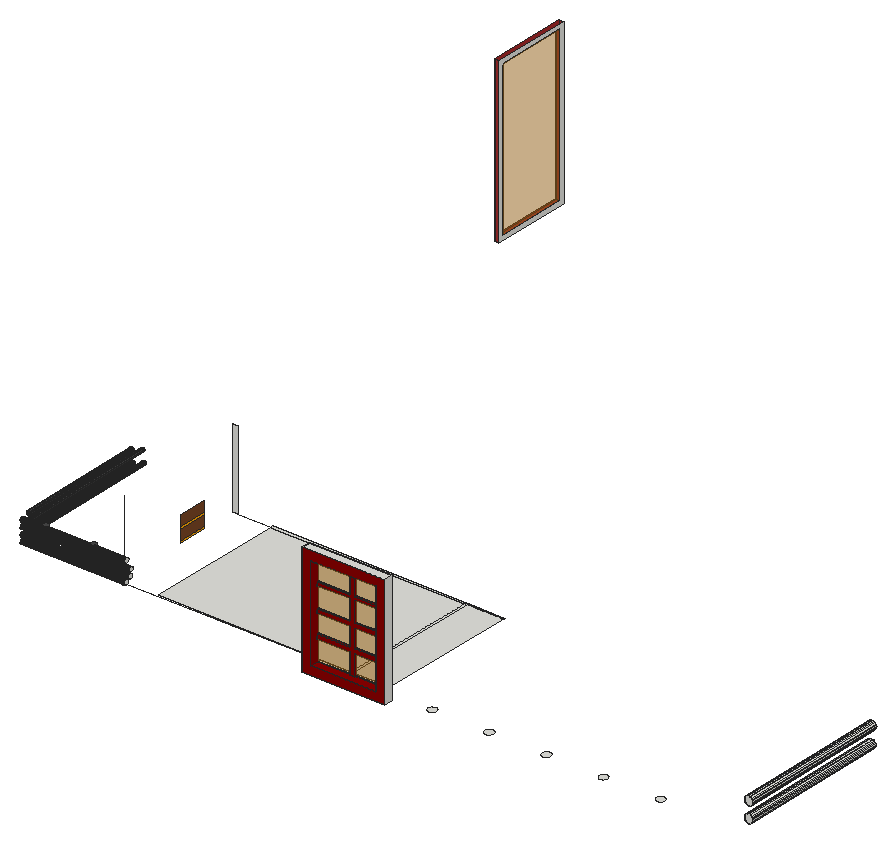
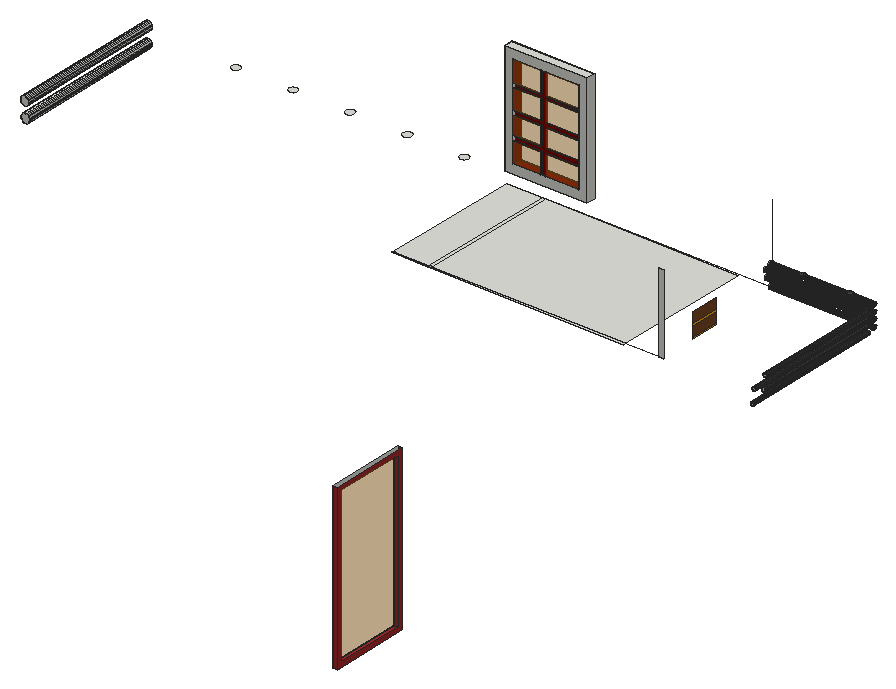
# SketchUp Ruby script. Lengths in inches.
U = 1.inch
M = Sketchup.active_model
def pt(a) = Geom::Point3d.new(a.map { |v| v * U })
def face(e, loops, mat)
  f = e.add_face(loops[0].map { |a| pt(a) })
  loops[1..].each { |l| e.add_face(l.map { |a| pt(a) }).erase! }
  f.material = f.back_material = mat if mat
  f
end
# faces: each face lists its corners as indices into pts; further lists are holes
def faces(e, pts, list, mat = nil) = list.each { |f| face(e, (f[0].is_a?(Array) ? f : [f]).map { |l| l.map { |i| pts[i] } }, mat) }
# xy, xz, yz: faces in a plane at the given z, y or x. An outline is a flat list of corners, or four numbers for a rectangle; further outlines are holes
def ring(l) = l.size == 4 ? [[l[0], l[1]], [l[2], l[1]], [l[2], l[3]], [l[0], l[3]]] : l.each_slice(2).to_a
def flat(e, list, mat, &to3) = list.each { |f| face(e, (f[0].is_a?(Array) ? f : [f]).map { |l| ring(l).map { |u, v| to3.(u, v) } }, mat) }
def xy(e, z, list, mat = nil) = flat(e, list, mat) { |x, y| [x, y, z] }
def xz(e, y, list, mat = nil) = flat(e, list, mat) { |x, z| [x, y, z] }
def yz(e, x, list, mat = nil) = flat(e, list, mat) { |y, z| [x, y, z] }
def lines(e, pts, list) = list.each { |a, b| e.add_line(pt(pts[a]), pt(pts[b])) }
# prism: a flat outline (further loops are holes) pulled along v
def prism(e, loops, v, mat = nil)
  f = face(e, loops, mat); d = Geom::Vector3d.new(v.map { |x| x * U })
  f.pushpull(f.normal.samedirection?(d) ? d.length : -d.length)
end
def box(e, o, s, mat = nil) = prism(e, [[o, [o[0] + s[0], o[1], o[2]], [o[0] + s[0], o[1] + s[1], o[2]], [o[0], o[1] + s[1], o[2]]]], [0, 0, s[2]], mat)
def at(x, y, z, deg = 0) = Geom::Transformation.translation(pt([x, y, z])) * Geom::Transformation.rotation(ORIGIN, Z_AXIS, deg.degrees)
def axes(o, x, y, z) = Geom::Transformation.new([*x, 0, *y, 0, *z, 0, *pt(o).to_a, 1])
def part(name) = M.definitions.add(name)
# library, detail: a bought-in or finely detailed component or shape, given as its bounding box
def library(name, o, s) = part(name).tap { |d| box(d.entities, o, s) }
def detail(e, o, s) = box(e.add_group.entities, o, s)
def put(e, d, t, mat = nil) = e.add_instance(d, t).tap { |i| i.material = mat if mat }
def group(e, t, mat = nil) = e.add_group.tap { |g| g.transformation = t; g.material = mat if mat }.entities
root = M.entities
M.materials.add("[0018_Brown]").color = [165, 42, 42]
M.materials.add("[0021_DarkRed]").color = [139, 0, 0]
M.materials.add("[0038_Orange]").color = [255, 165, 0]
M.materials.add("[0137_Black]").color = [71, 71, 71]
M.materials.add("[Translucent Glass Gray]").color = [191, 123, 24]
M.materials["[Translucent Glass Gray]"].alpha = 0.5
M.materials.add("[Wood Veneer 01]").color = [120, 70, 37]
prism(root,[[[502.06,26.4375,435.45],[501.3,26.4375,435.55],[500.54,26.4375,435.45],[499.83,26.4375,435.16],[499.22,26.4375,434.69],[498.75,26.4375,434.08],[498.46,26.4375,433.375],[498.36,26.4375,432.62],[498.46,26.4375,431.85],[498.75,26.4375,431.15],[499.22,26.4375,430.54],[499.83,26.4375,430.07],[500.54,26.4375,429.78],[501.3,26.4375,429.68],[502.06,26.4375,429.78],[502.77,26.4375,430.07],[503.375,26.4375,430.54],[503.84,26.4375,431.15],[504.13,26.4375,431.85],[504.23,26.4375,432.62],[504.13,26.4375,433.375],[503.84,26.4375,434.08],[503.375,26.4375,434.69],[502.77,26.4375,435.16]]],[0,102.5,0])
prism(root,[[[502.06,26.4375,446.2],[501.3,26.4375,446.3],[500.54,26.4375,446.2],[499.83,26.4375,445.91],[499.22,26.4375,445.44],[498.75,26.4375,444.83],[498.46,26.4375,444.125],[498.36,26.4375,443.37],[498.46,26.4375,442.6],[498.75,26.4375,441.9],[499.22,26.4375,441.29],[499.83,26.4375,440.82],[500.54,26.4375,440.53],[501.3,26.4375,440.43],[502.06,26.4375,440.53],[502.77,26.4375,440.82],[503.375,26.4375,441.29],[503.84,26.4375,441.9],[504.13,26.4375,442.6],[504.23,26.4375,443.37],[504.13,26.4375,444.125],[503.84,26.4375,444.83],[503.375,26.4375,445.44],[502.77,26.4375,445.91]]],[0,103.125,0])
xy(root,429.83,[[8.875,428.78,11.875,482.72]],"[0018_Brown]")
xy(root,429.92,[[217.92,6.1875,273.55,12.1875]])
xy(root,429.99,[[264.04,22.25,264.91,116.51,240.73,116.73,239.85,22.47],[239.85,22.47,237.79,22.49,238.66,116.75,240.73,116.73],[237.79,22.49,238.66,116.75,240.73,116.75,240.73,117.16,238.67,117.18,238.66,116.75,108.66,116.75,107.8,23.69],[264.91,116.51,264.91,116.75,240.73,116.75,240.73,116.73],[240.73,116.73,240.73,116.75,238.66,116.75],
  [108.66,116.75,238.66,116.75,238.67,117.18,108.67,118.38],[240.73,116.75,264.91,116.75,264.92,116.9375,240.73,117.16]])
xy(root,431.18,[[297.64,12.9375,298.33,13.03,298.98,13.3,299.54,13.72,299.96,14.28,300.23,14.93,300.32,15.625,300.23,16.32,299.97,16.97,299.54,17.53,298.98,17.95,298.33,18.22,297.64,18.3125,296.94,18.22,296.29,17.95,295.74,17.53,295.31,16.97,295.04,16.32,294.95,15.625,295.04,14.93,295.31,14.28,295.74,13.73,296.29,13.3,296.94,13.03],[335.89,12.9375,336.58,13.03,337.23,13.3,337.79,13.72,338.21,14.28,338.48,14.93,338.57,15.625,338.48,16.32,338.22,16.97,337.79,17.53,337.23,17.95,336.58,18.22,335.89,18.3125,335.19,18.22,334.54,17.95,333.99,17.53,333.56,16.97,333.29,16.32,333.2,15.625,333.29,14.93,333.56,14.28,333.99,13.73,334.54,13.3,335.19,13.03],[374.14,12.9375,374.83,13.03,375.48,13.3,376.04,13.72,376.46,14.28,376.73,14.93,376.82,15.625,376.73,16.32,376.47,16.97,376.04,17.53,375.48,17.95,374.83,18.22,374.14,18.3125,373.44,18.22,372.79,17.95,372.24,17.53,371.81,16.97,371.54,16.32,371.45,15.625,371.54,14.93,371.81,14.28,372.24,13.73,372.79,13.3,373.44,13.03],[412.39,12.9375,413.08,13.03,413.73,13.3,414.29,13.72,414.71,14.28,414.98,14.93,415.07,15.625,414.98,16.32,414.72,16.97,414.29,17.53,413.73,17.95,413.08,18.22,412.39,18.3125,411.69,18.22,411.04,17.95,410.49,17.53,410.06,16.97,409.79,16.32,409.7,15.625,409.79,14.93,410.06,14.28,410.49,13.73,411.04,13.3,411.69,13.03],[450.64,12.9375,451.33,13.03,451.98,13.3,452.54,13.72,452.96,14.28,453.23,14.93,453.32,15.625,453.23,16.32,452.97,16.97,452.54,17.53,451.98,17.95,451.33,18.22,450.64,18.3125,449.94,18.22,449.29,17.95,448.74,17.53,448.31,16.97,448.04,16.32,447.95,15.625,448.04,14.93,448.31,14.28,448.74,13.73,449.29,13.3,449.94,13.03]])
xy(root,432.83,[[8.875,431.78,11.875,479.72]],"[0018_Brown]")
xy(root,435.86,[[245.74,11.1875,249.17,12.1875]])
xy(root,435.86,[[223.87,6.1875,267.6,6.1875,267.6,12.1875,249.17,12.1875,249.17,11.1875,245.74,11.1875,245.74,12.1875,223.87,12.1875]],"[0021_DarkRed]")
xy(root,446.03,[[32.63,21.64,33.02,21.69,33.38,21.84,33.7,22.08,33.93,22.39,34.08,22.75,34.13,23.14,34.08,23.53,33.93,23.89,33.7,24.2,33.38,24.44,33.02,24.59,32.63,24.64,32.25,24.59,31.88,24.44,31.57,24.2,31.34,23.89,31.1875,23.53,31.13,23.14,31.1875,22.75,31.34,22.39,31.57,22.08,31.88,21.84,32.25,21.69],[64.82,21.64,65.21,21.69,65.57,21.84,65.88,22.08,66.12,22.39,66.27,22.75,66.32,23.14,66.27,23.53,66.12,23.89,65.88,24.2,65.57,24.44,65.21,24.59,64.82,24.64,64.43,24.59,64.07,24.44,63.76,24.2,63.52,23.89,63.375,23.53,63.32,23.14,63.375,22.75,63.52,22.39,63.76,22.08,64.07,21.84,64.43,21.69]],"[0137_Black]")
xy(root,449.8,[[223.87,11.1875,245.74,12.1875],[249.17,11.1875,267.6,12.1875]],"[0021_DarkRed]")
xy(root,453.02,[[223.87,11.1875,245.74,12.1875],[249.17,11.1875,267.6,12.1875]],"[0021_DarkRed]")
xy(root,465.24,[[223.87,11.1875,245.74,12.1875],[249.17,11.1875,267.6,12.1875]],"[0021_DarkRed]")
xy(root,468.1,[[223.87,11.1875,245.74,12.1875],[249.17,11.1875,267.6,12.1875]],"[0021_DarkRed]")
xy(root,481.95,[[223.87,11.1875,245.74,12.1875],[249.17,11.1875,267.6,12.1875]],"[0021_DarkRed]")
xy(root,484,[[223.87,11.1875,245.74,12.1875],[249.17,11.1875,267.6,12.1875]],"[0021_DarkRed]")
xy(root,499.09,[[245.74,11.1875,249.17,12.1875]])
xy(root,499.09,[[223.87,6.1875,223.87,12.1875,245.74,12.1875,245.74,11.1875,249.17,11.1875,249.17,12.1875,267.6,12.1875,267.6,6.1875]],"[0021_DarkRed]")
xy(root,505.04,[[217.92,6.1875,273.55,12.1875]])
xz(root,6.1875,[[[217.92,429.92,273.55,505.04],[223.87,435.86,267.6,499.09]]],"[0021_DarkRed]")
xz(root,11.1875,[[245.74,435.86,249.17,435.86,249.17,449.8,267.6,449.8,267.6,453.02,249.17,453.02,249.17,465.24,267.6,465.24,267.6,468.1,249.17,468.1,249.17,481.95,267.6,481.95,267.6,484,249.17,484,249.17,499.09,245.74,499.09,245.74,484,223.87,484,223.87,481.95,245.74,481.95,245.74,468.1,223.87,468.1,223.87,465.24,245.74,465.24,245.74,453.02,223.87,453.02,223.87,449.8,245.74,449.8]],"[0021_DarkRed]")
xz(root,12.1875,[[[217.92,429.92,273.55,505.04],[223.87,435.86,267.6,499.09]]])
xz(root,12.1875,[[223.87,435.86,245.74,449.8],[249.17,435.86,267.6,449.8],[223.87,453.02,245.74,465.24],[249.17,453.02,267.6,465.24],[223.87,468.1,245.74,481.95],
  [249.17,468.1,267.6,481.95],[223.87,484,245.74,499.09],[249.17,484,267.6,499.09]],"[Translucent Glass Gray]")
xz(root,116.75,[[82.85,429.99,86.03,483]])
xz(root,117.125,[[14.9,442.72,14.6,442.76,14.3125,442.875,14.07,443.0625,13.875,443.31,13.76,443.6,13.72,443.9,13.76,444.21,13.875,444.5,14.07,444.74,14.3125,444.93,14.6,445.05,14.9,445.09,15.21,445.05,15.5,444.93,15.74,444.74,15.93,444.5,16.05,444.21,16.09,443.9,16.05,443.6,15.93,443.31,15.74,443.0625,15.5,442.875,15.21,442.76]])
xz(root,118.0625,[[14.9,434.22,14.6,434.26,14.3125,434.375,14.07,434.5625,13.875,434.81,13.76,435.1,13.72,435.4,13.76,435.71,13.875,436,14.07,436.24,14.3125,436.43,14.6,436.55,14.9,436.59,15.21,436.55,15.5,436.43,15.74,436.24,15.93,436,16.05,435.71,16.09,435.4,16.05,435.1,15.93,434.81,15.74,434.5625,15.5,434.375,15.21,434.26]])
xz(root,126.3125,[[14.9,438.47,14.6,438.51,14.3125,438.625,14.07,438.8125,13.875,439.06,13.76,439.35,13.72,439.65,13.76,439.96,13.875,440.25,14.07,440.49,14.3125,440.68,14.6,440.8,14.9,440.84,15.21,440.8,15.5,440.68,15.74,440.49,15.93,440.25,16.05,439.96,16.09,439.65,16.05,439.35,15.93,439.06,15.74,438.8125,15.5,438.625,15.21,438.51]])
xz(root,127.5625,[[14.9,429.97,14.6,430.01,14.3125,430.125,14.07,430.3125,13.875,430.56,13.76,430.85,13.72,431.15,13.76,431.46,13.875,431.75,14.07,431.99,14.3125,432.18,14.6,432.3,14.9,432.34,15.21,432.3,15.5,432.18,15.74,431.99,15.93,431.75,16.05,431.46,16.09,431.15,16.05,430.85,15.93,430.56,15.74,430.3125,15.5,430.125,15.21,430.01]])
xz(root,428.78,[[8.875,429.83,11.875,539.15]],"[0018_Brown]")
xz(root,431.78,[[8.875,432.83,11.875,536.15]],"[0018_Brown]")
xz(root,479.72,[[8.875,432.83,11.875,536.15]],"[0018_Brown]")
xz(root,482.72,[[8.875,429.83,11.875,539.15]],"[0018_Brown]")
yz(root,8.875,[[[428.78,429.83,482.72,539.15],[431.78,432.83,479.72,536.15]]],"[0018_Brown]")
yz(root,11.875,[[[428.78,429.83,482.72,539.15],[431.78,432.83,479.72,536.15]]])
yz(root,11.875,[[431.78,432.83,479.72,536.15]],"[Translucent Glass Gray]")
yz(root,82.85,[[73.09,430.75,92.21,431.86],[73.09,439.0625,92.21,440.18]],"[0038_Orange]")
yz(root,82.85,[[73.09,431.86,92.21,439.0625],[73.09,440.18,92.21,447.375]],"[Wood Veneer 01]")
yz(root,86.9375,[[22.6,429.27,22.96,429.3125,23.29,429.45,23.58,429.67,23.8,429.96,23.93,430.29,23.98,430.64,23.93,431,23.8,431.33,23.58,431.61,23.29,431.83,22.96,431.97,22.6,432.02,22.25,431.97,21.92,431.83,21.63,431.61,21.41,431.33,21.28,431,21.23,430.64,21.28,430.29,21.41,429.96,21.63,429.67,21.92,429.45,22.25,429.3125]])
yz(root,87.1875,[[22.6,442.77,22.96,442.8125,23.29,442.95,23.58,443.17,23.8,443.46,23.93,443.79,23.98,444.14,23.93,444.5,23.8,444.83,23.58,445.11,23.29,445.33,22.96,445.47,22.6,445.52,22.25,445.47,21.92,445.33,21.63,445.11,21.41,444.83,21.28,444.5,21.23,444.14,21.28,443.79,21.41,443.46,21.63,443.17,21.92,442.95,22.25,442.8125]])
yz(root,89.5,[[22.6,433.77,22.96,433.8125,23.29,433.95,23.58,434.17,23.8,434.46,23.93,434.79,23.98,435.14,23.93,435.5,23.8,435.83,23.58,436.11,23.29,436.33,22.96,436.47,22.6,436.52,22.25,436.47,21.92,436.33,21.63,436.11,21.41,435.83,21.28,435.5,21.23,435.14,21.28,434.79,21.41,434.46,21.63,434.17,21.92,433.95,22.25,433.8125]])
yz(root,90.1875,[[22.6,438.27,22.96,438.3125,23.29,438.45,23.58,438.67,23.8,438.96,23.93,439.29,23.98,439.64,23.93,440,23.8,440.33,23.58,440.61,23.29,440.83,22.96,440.97,22.6,441.02,22.25,440.97,21.92,440.83,21.63,440.61,21.41,440.33,21.28,440,21.23,439.64,21.28,439.29,21.41,438.96,21.63,438.67,21.92,438.45,22.25,438.3125]])
yz(root,217.92,[[6.1875,429.92,12.1875,505.04]])
yz(root,223.87,[[11.1875,449.8,12.1875,453.02],[11.1875,465.24,12.1875,468.1],[11.1875,481.95,12.1875,484]])
yz(root,223.87,[[6.1875,435.86,12.1875,435.86,12.1875,449.8,11.1875,449.8,11.1875,453.02,12.1875,453.02,12.1875,465.24,11.1875,465.24,11.1875,468.1,12.1875,468.1,12.1875,481.95,11.1875,481.95,11.1875,484,12.1875,484,12.1875,499.09,6.1875,499.09]],"[0021_DarkRed]")
yz(root,245.74,[[11.1875,435.86,12.1875,449.8],[11.1875,453.02,12.1875,465.24],[11.1875,468.1,12.1875,481.95],[11.1875,484,12.1875,499.09]],"[0021_DarkRed]")
yz(root,249.17,[[11.1875,435.86,12.1875,449.8],[11.1875,453.02,12.1875,465.24],[11.1875,468.1,12.1875,481.95],[11.1875,484,12.1875,499.09]],"[0021_DarkRed]")
yz(root,267.6,[[11.1875,449.8,12.1875,453.02],[11.1875,465.24,12.1875,468.1],[11.1875,481.95,12.1875,484]])
yz(root,267.6,[[6.1875,435.86,6.1875,499.09,12.1875,499.09,12.1875,484,11.1875,484,11.1875,481.95,12.1875,481.95,12.1875,468.1,11.1875,468.1,11.1875,465.24,12.1875,465.24,12.1875,453.02,11.1875,453.02,11.1875,449.8,12.1875,449.8,12.1875,435.86]],"[0021_DarkRed]")
yz(root,273.55,[[6.1875,429.92,12.1875,505.04]])
p = [[16.875,21.92,429.45],[16.875,22.25,429.3125],[86.9375,22.25,429.3125],[86.9375,21.92,429.45],[16.875,22.6,429.27],[86.9375,22.6,429.27],
  [16.875,22.96,429.3125],[86.9375,22.96,429.3125],[16.875,23.29,429.45],[86.9375,23.29,429.45],[16.875,21.63,429.67],[86.9375,21.63,429.67],
  [16.875,23.58,429.67],[86.9375,23.58,429.67],[16.875,21.41,429.96],[86.9375,21.41,429.96],[16.875,23.8,429.96],[86.9375,23.8,429.96],
  [16.875,21.28,430.29],[86.9375,21.28,430.29],[16.875,23.93,430.29],[86.9375,23.93,430.29],[14.6,30.25,430.01],[14.3125,30.25,430.125],
  [14.3125,127.5625,430.125],[14.6,127.5625,430.01],[14.9,30.25,429.97],[14.9,127.5625,429.97],[15.21,30.25,430.01],[15.21,127.5625,430.01],
  [15.5,30.25,430.125],[15.5,127.5625,430.125],[14.07,30.25,430.3125],[14.07,127.5625,430.3125],[15.74,30.25,430.3125],[15.74,127.5625,430.3125],
  [16.875,21.23,430.64],[86.9375,21.23,430.64],[16.875,23.98,430.64],[86.9375,23.98,430.64],[13.875,30.25,430.56],[13.875,127.5625,430.56],
  [15.93,30.25,430.56],[15.93,127.5625,430.56],[16.875,21.28,431],[86.9375,21.28,431],[16.875,23.93,431],[86.9375,23.93,431],
  [13.76,30.25,430.85],[13.76,127.5625,430.85],[16.05,30.25,430.85],[16.05,127.5625,430.85],[13.72,30.25,431.15],[13.72,127.5625,431.15],
  [16.09,30.25,431.15],[16.09,127.5625,431.15],[16.875,21.41,431.33],[86.9375,21.41,431.33],[16.875,23.8,431.33],[86.9375,23.8,431.33],
  [13.76,30.25,431.46],[13.76,127.5625,431.46],[16.05,30.25,431.46],[16.05,127.5625,431.46],[16.875,21.63,431.61],[86.9375,21.63,431.61],
  [16.875,23.58,431.61],[86.9375,23.58,431.61],[13.875,30.25,431.75],[13.875,127.5625,431.75],[15.93,30.25,431.75],[15.93,127.5625,431.75],
  [16.875,21.92,431.83],[86.9375,21.92,431.83],[16.875,23.29,431.83],[86.9375,23.29,431.83],[14.07,30.25,431.99],[14.07,127.5625,431.99],
  [15.74,30.25,431.99],[15.74,127.5625,431.99],[16.875,22.25,431.97],[86.9375,22.25,431.97],[16.875,22.96,431.97],[86.9375,22.96,431.97],
  [16.875,22.6,432.02],[86.9375,22.6,432.02],[14.3125,30.25,432.18],[14.3125,127.5625,432.18],[15.5,30.25,432.18],[15.5,127.5625,432.18],
  [14.6,30.25,432.3],[14.6,127.5625,432.3],[15.21,30.25,432.3],[15.21,127.5625,432.3],[14.9,30.25,432.34],[14.9,127.5625,432.34],
  [16.875,21.92,433.95],[16.875,22.25,433.8125],[89.5,22.25,433.8125],[89.5,21.92,433.95],[16.875,22.6,433.77],[89.5,22.6,433.77],
  [16.875,22.96,433.8125],[89.5,22.96,433.8125],[16.875,23.29,433.95],[89.5,23.29,433.95],[16.875,21.63,434.17],[89.5,21.63,434.17],
  [16.875,23.58,434.17],[89.5,23.58,434.17],[16.875,21.41,434.46],[89.5,21.41,434.46],[16.875,23.8,434.46],[89.5,23.8,434.46],
  [14.9,30.25,434.22],[14.6,30.25,434.26],[14.6,118.0625,434.26],[14.9,118.0625,434.22],[15.21,30.25,434.26],[15.21,118.0625,434.26],
  [14.3125,30.25,434.375],[14.3125,118.0625,434.375],[15.5,30.25,434.375],[15.5,118.0625,434.375],[14.07,30.25,434.5625],[14.07,118.0625,434.5625],
  [15.74,30.25,434.5625],[15.74,118.0625,434.5625],[16.875,21.28,434.79],[89.5,21.28,434.79],[16.875,23.93,434.79],[89.5,23.93,434.79],
  [13.875,30.25,434.81],[13.875,118.0625,434.81],[15.93,30.25,434.81],[15.93,118.0625,434.81],[16.875,21.23,435.14],[89.5,21.23,435.14],
  [16.875,23.98,435.14],[89.5,23.98,435.14],[13.76,30.25,435.1],[13.76,118.0625,435.1],[16.05,30.25,435.1],[16.05,118.0625,435.1],
  [16.875,21.28,435.5],[89.5,21.28,435.5],[16.875,23.93,435.5],[89.5,23.93,435.5],[13.72,30.25,435.4],[13.72,118.0625,435.4],
  [16.09,30.25,435.4],[16.09,118.0625,435.4],[13.76,30.25,435.71],[13.76,118.0625,435.71],[16.05,30.25,435.71],[16.05,118.0625,435.71],
  [16.875,21.41,435.83],[89.5,21.41,435.83],[16.875,23.8,435.83],[89.5,23.8,435.83],[13.875,30.25,436],[13.875,118.0625,436],
  [15.93,30.25,436],[15.93,118.0625,436],[16.875,21.63,436.11],[89.5,21.63,436.11],[16.875,23.58,436.11],[89.5,23.58,436.11],
  [14.07,30.25,436.24],[14.07,118.0625,436.24],[15.74,30.25,436.24],[15.74,118.0625,436.24],[16.875,21.92,436.33],[89.5,21.92,436.33],
  [16.875,23.29,436.33],[89.5,23.29,436.33],[14.3125,30.25,436.43],[14.3125,118.0625,436.43],[15.5,30.25,436.43],[15.5,118.0625,436.43],
  [16.875,22.25,436.47],[89.5,22.25,436.47],[16.875,22.96,436.47],[89.5,22.96,436.47],[14.6,30.25,436.55],[14.6,118.0625,436.55],
  [15.21,30.25,436.55],[15.21,118.0625,436.55],[16.875,22.6,436.52],[89.5,22.6,436.52],[14.9,30.25,436.59],[14.9,118.0625,436.59],
  [16.875,21.92,438.45],[16.875,22.25,438.3125],[90.1875,22.25,438.3125],[90.1875,21.92,438.45],[16.875,22.6,438.27],[90.1875,22.6,438.27],
  [16.875,22.96,438.3125],[90.1875,22.96,438.3125],[16.875,23.29,438.45],[90.1875,23.29,438.45],[16.875,21.63,438.67],[90.1875,21.63,438.67],
  [16.875,23.58,438.67],[90.1875,23.58,438.67],[14.6,30.25,438.51],[14.3125,30.25,438.625],[14.3125,126.3125,438.625],[14.6,126.3125,438.51],
  [14.9,30.25,438.47],[14.9,126.3125,438.47],[15.21,30.25,438.51],[15.21,126.3125,438.51],[15.5,30.25,438.625],[15.5,126.3125,438.625],
  [14.07,30.25,438.8125],[14.07,126.3125,438.8125],[15.74,30.25,438.8125],[15.74,126.3125,438.8125],[16.875,21.41,438.96],[90.1875,21.41,438.96],
  [16.875,23.8,438.96],[90.1875,23.8,438.96],[13.875,30.25,439.06],[13.875,126.3125,439.06],[15.93,30.25,439.06],[15.93,126.3125,439.06],
  [16.875,21.28,439.29],[90.1875,21.28,439.29],[16.875,23.93,439.29],[90.1875,23.93,439.29],[13.76,30.25,439.35],[13.76,126.3125,439.35],
  [16.05,30.25,439.35],[16.05,126.3125,439.35],[16.875,21.23,439.64],[90.1875,21.23,439.64],[16.875,23.98,439.64],[90.1875,23.98,439.64],
  [13.72,30.25,439.65],[13.72,126.3125,439.65],[16.09,30.25,439.65],[16.09,126.3125,439.65],[16.875,21.28,440],[90.1875,21.28,440],
  [16.875,23.93,440],[90.1875,23.93,440],[13.76,30.25,439.96],[13.76,126.3125,439.96],[16.05,30.25,439.96],[16.05,126.3125,439.96],
  [16.875,21.41,440.33],[90.1875,21.41,440.33],[16.875,23.8,440.33],[90.1875,23.8,440.33],[13.875,30.25,440.25],[13.875,126.3125,440.25],
  [15.93,30.25,440.25],[15.93,126.3125,440.25],[14.07,30.25,440.49],[14.07,126.3125,440.49],[15.74,30.25,440.49],[15.74,126.3125,440.49],
  [16.875,21.63,440.61],[90.1875,21.63,440.61],[16.875,23.58,440.61],[90.1875,23.58,440.61],[14.3125,30.25,440.68],[14.3125,126.3125,440.68],
  [15.5,30.25,440.68],[15.5,126.3125,440.68],[16.875,21.92,440.83],[90.1875,21.92,440.83],[16.875,23.29,440.83],[90.1875,23.29,440.83],
  [14.6,30.25,440.8],[14.6,126.3125,440.8],[15.21,30.25,440.8],[15.21,126.3125,440.8],[16.875,22.25,440.97],[90.1875,22.25,440.97],
  [16.875,22.96,440.97],[90.1875,22.96,440.97],[14.9,30.25,440.84],[14.9,126.3125,440.84],[16.875,22.6,441.02],[90.1875,22.6,441.02],
  [14.9,30.25,442.72],[14.6,30.25,442.76],[14.6,117.125,442.76],[14.9,117.125,442.72],[15.21,30.25,442.76],[15.21,117.125,442.76],
  [16.875,21.92,442.95],[16.875,22.25,442.8125],[87.1875,22.25,442.8125],[87.1875,21.92,442.95],[16.875,22.6,442.77],[87.1875,22.6,442.77],
  [16.875,22.96,442.8125],[87.1875,22.96,442.8125],[16.875,23.29,442.95],[87.1875,23.29,442.95],[14.3125,30.25,442.875],[14.3125,117.125,442.875],
  [15.5,30.25,442.875],[15.5,117.125,442.875],[14.07,30.25,443.0625],[14.07,117.125,443.0625],[15.74,30.25,443.0625],[15.74,117.125,443.0625],
  [16.875,21.63,443.17],[87.1875,21.63,443.17],[16.875,23.58,443.17],[87.1875,23.58,443.17],[13.875,30.25,443.31],[13.875,117.125,443.31],
  [15.93,30.25,443.31],[15.93,117.125,443.31],[16.875,21.41,443.46],[87.1875,21.41,443.46],[16.875,23.8,443.46],[87.1875,23.8,443.46],
  [13.76,30.25,443.6],[13.76,117.125,443.6],[16.05,30.25,443.6],[16.05,117.125,443.6],[16.875,21.28,443.79],[87.1875,21.28,443.79],
  [16.875,23.93,443.79],[87.1875,23.93,443.79],[13.72,30.25,443.9],[13.72,117.125,443.9],[16.09,30.25,443.9],[16.09,117.125,443.9],
  [16.875,21.23,444.14],[87.1875,21.23,444.14],[16.875,23.98,444.14],[87.1875,23.98,444.14],[13.76,30.25,444.21],[13.76,117.125,444.21],
  [16.05,30.25,444.21],[16.05,117.125,444.21],[16.875,21.28,444.5],[87.1875,21.28,444.5],[16.875,23.93,444.5],[87.1875,23.93,444.5],
  [13.875,30.25,444.5],[13.875,117.125,444.5],[15.93,30.25,444.5],[15.93,117.125,444.5],[16.875,21.41,444.83],[87.1875,21.41,444.83],
  [16.875,23.8,444.83],[87.1875,23.8,444.83],[14.07,30.25,444.74],[14.07,117.125,444.74],[15.74,30.25,444.74],[15.74,117.125,444.74],
  [14.3125,30.25,444.93],[14.3125,117.125,444.93],[15.5,30.25,444.93],[15.5,117.125,444.93],[16.875,21.63,445.11],[87.1875,21.63,445.11],
  [16.875,23.58,445.11],[87.1875,23.58,445.11],[14.6,30.25,445.05],[14.6,117.125,445.05],[15.21,30.25,445.05],[15.21,117.125,445.05],
  [16.875,21.92,445.33],[87.1875,21.92,445.33],[16.875,23.29,445.33],[87.1875,23.29,445.33],[14.9,30.25,445.09],[14.9,117.125,445.09],
  [16.875,22.25,445.47],[87.1875,22.25,445.47],[16.875,22.96,445.47],[87.1875,22.96,445.47],[16.875,22.6,445.52],[87.1875,22.6,445.52],
  [238.66,22.0625,429.99],[211.73,22.0625,429.99],[108.66,116.75,429.99],[86.03,116.75,429.99],[86.03,22.0625,429.99],[86.03,22.0625,483]]
faces(root,p,[[0,1,2,3],[1,4,5,2],[4,6,7,5],[6,8,9,7],[10,0,3,11],[8,12,13,9],[14,10,11,15],[12,16,17,13],
  [18,14,15,19],[16,20,21,17],[22,23,24,25],[26,22,25,27],[28,26,27,29],[30,28,29,31],[23,32,33,24],[34,30,31,35],
  [36,18,19,37],[20,38,39,21],[32,40,41,33],[42,34,35,43],[44,36,37,45],[38,46,47,39],[40,48,49,41],[50,42,43,51],
  [48,52,53,49],[54,50,51,55],[56,44,45,57],[46,58,59,47],[52,60,61,53],[62,54,55,63],[64,56,57,65],[58,66,67,59],
  [60,68,69,61],[70,62,63,71],[72,64,65,73],[66,74,75,67],[68,76,77,69],[78,70,71,79],[80,72,73,81],[74,82,83,75],
  [84,80,81,85],[82,84,85,83],[76,86,87,77],[88,78,79,89],[86,90,91,87],[92,88,89,93],[90,94,95,91],[94,92,93,95],
  [96,97,98,99],[97,100,101,98],[100,102,103,101],[102,104,105,103],[106,96,99,107],[104,108,109,105],[110,106,107,111],[108,112,113,109],
  [114,115,116,117],[118,114,117,119],[115,120,121,116],[122,118,119,123],[120,124,125,121],[126,122,123,127],[128,110,111,129],[112,130,131,113],
  [124,132,133,125],[134,126,127,135],[136,128,129,137],[130,138,139,131],[132,140,141,133],[142,134,135,143],[144,136,137,145],[138,146,147,139],
  [140,148,149,141],[150,142,143,151],[148,152,153,149],[154,150,151,155],[156,144,145,157],[146,158,159,147],[152,160,161,153],[162,154,155,163],
  [164,156,157,165],[158,166,167,159],[160,168,169,161],[170,162,163,171],[172,164,165,173],[166,174,175,167],[168,176,177,169],[178,170,171,179],
  [180,172,173,181],[174,182,183,175],[176,184,185,177],[186,178,179,187],[188,180,181,189],[182,188,189,183],[184,190,191,185],[190,186,187,191],
  [192,193,194,195],[193,196,197,194],[196,198,199,197],[198,200,201,199],[202,192,195,203],[200,204,205,201],[206,207,208,209],[210,206,209,211],
  [212,210,211,213],[214,212,213,215],[207,216,217,208],[218,214,215,219],[220,202,203,221],[204,222,223,205],[216,224,225,217],[226,218,219,227],
  [228,220,221,229],[222,230,231,223],[224,232,233,225],[234,226,227,235],[236,228,229,237],[230,238,239,231],[232,240,241,233],[242,234,235,243],
  [244,236,237,245],[238,246,247,239],[240,248,249,241],[250,242,243,251],[252,244,245,253],[246,254,255,247],[248,256,257,249],[258,250,251,259],
  [256,260,261,257],[262,258,259,263],[264,252,253,265],[254,266,267,255],[260,268,269,261],[270,262,263,271],[272,264,265,273],[266,274,275,267],
  [268,276,277,269],[278,270,271,279],[280,272,273,281],[274,282,283,275],[276,284,285,277],[284,278,279,285],[286,280,281,287],[282,286,287,283],
  [288,289,290,291],[292,288,291,293],[294,295,296,297],[295,298,299,296],[298,300,301,299],[300,302,303,301],[289,304,305,290],[306,292,293,307],
  [304,308,309,305],[310,306,307,311],[312,294,297,313],[302,314,315,303],[308,316,317,309],[318,310,311,319],[320,312,313,321],[314,322,323,315],
  [316,324,325,317],[326,318,319,327],[328,320,321,329],[322,330,331,323],[324,332,333,325],[334,326,327,335],[336,328,329,337],[330,338,339,331],
  [332,340,341,333],[342,334,335,343],[344,336,337,345],[338,346,347,339],[340,348,349,341],[350,342,343,351],[352,344,345,353],[346,354,355,347],
  [348,356,357,349],[358,350,351,359],[356,360,361,357],[362,358,359,363],[364,352,353,365],[354,366,367,355],[360,368,369,361],[370,362,363,371],
  [372,364,365,373],[366,374,375,367],[368,376,377,369],[376,370,371,377],[378,372,373,379],[374,380,381,375],[382,378,379,383],[380,382,383,381]],"[0137_Black]")
lines(root,p,[[384,385],[386,387],[388,389],[385,388]])
